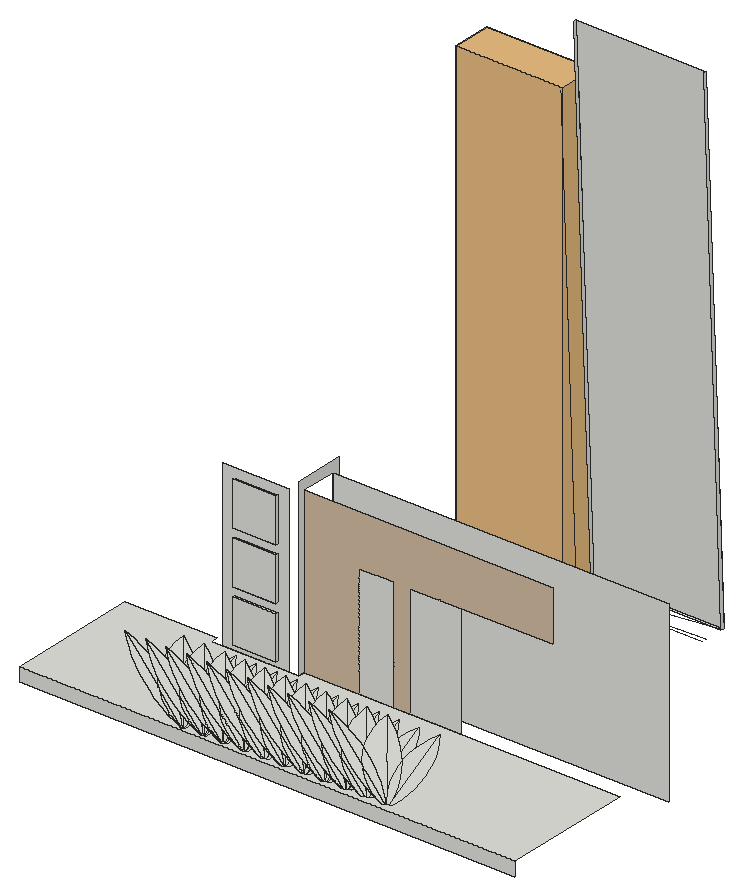
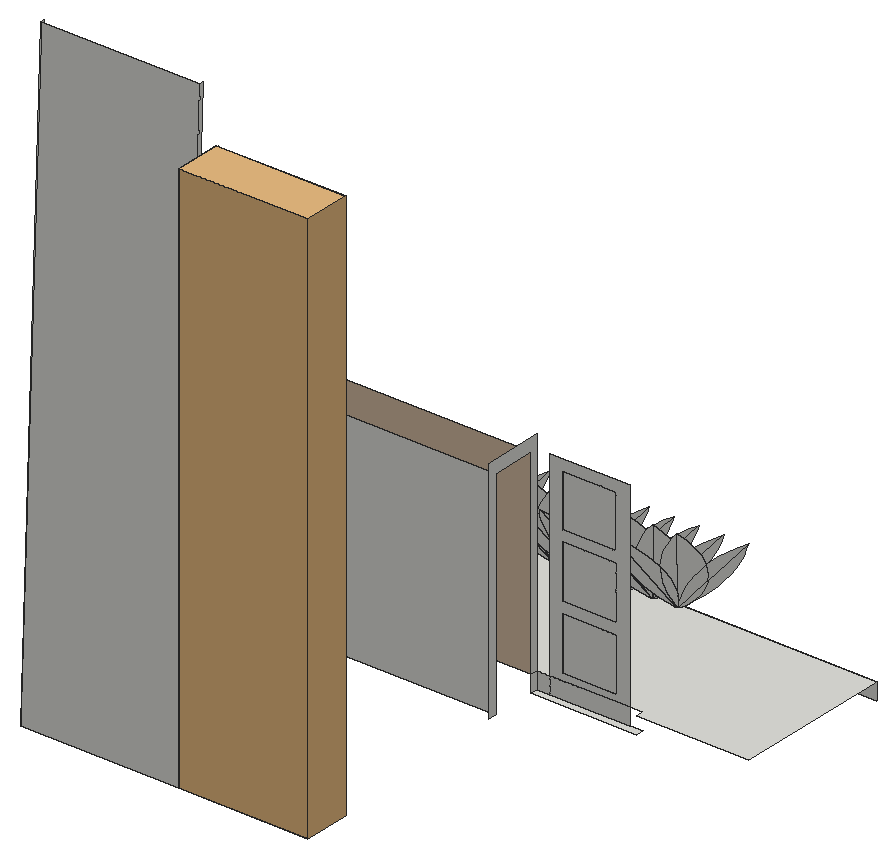
# SketchUp Ruby script. Lengths in inches.
U = 1.inch
M = Sketchup.active_model
def pt(a) = Geom::Point3d.new(a.map { |v| v * U })
def face(e, loops, mat)
  f = e.add_face(loops[0].map { |a| pt(a) })
  loops[1..].each { |l| e.add_face(l.map { |a| pt(a) }).erase! }
  f.material = f.back_material = mat if mat
  f
end
# faces: each face lists its corners as indices into pts; further lists are holes
def faces(e, pts, list, mat = nil) = list.each { |f| face(e, (f[0].is_a?(Array) ? f : [f]).map { |l| l.map { |i| pts[i] } }, mat) }
# xy, xz, yz: faces in a plane at the given z, y or x. An outline is a flat list of corners, or four numbers for a rectangle; further outlines are holes
def ring(l) = l.size == 4 ? [[l[0], l[1]], [l[2], l[1]], [l[2], l[3]], [l[0], l[3]]] : l.each_slice(2).to_a
def flat(e, list, mat, &to3) = list.each { |f| face(e, (f[0].is_a?(Array) ? f : [f]).map { |l| ring(l).map { |u, v| to3.(u, v) } }, mat) }
def xy(e, z, list, mat = nil) = flat(e, list, mat) { |x, y| [x, y, z] }
def xz(e, y, list, mat = nil) = flat(e, list, mat) { |x, z| [x, y, z] }
def yz(e, x, list, mat = nil) = flat(e, list, mat) { |y, z| [x, y, z] }
def lines(e, pts, list) = list.each { |a, b| e.add_line(pt(pts[a]), pt(pts[b])) }
# prism: a flat outline (further loops are holes) pulled along v
def prism(e, loops, v, mat = nil)
  f = face(e, loops, mat); d = Geom::Vector3d.new(v.map { |x| x * U })
  f.pushpull(f.normal.samedirection?(d) ? d.length : -d.length)
end
def box(e, o, s, mat = nil) = prism(e, [[o, [o[0] + s[0], o[1], o[2]], [o[0] + s[0], o[1] + s[1], o[2]], [o[0], o[1] + s[1], o[2]]]], [0, 0, s[2]], mat)
def at(x, y, z, deg = 0) = Geom::Transformation.translation(pt([x, y, z])) * Geom::Transformation.rotation(ORIGIN, Z_AXIS, deg.degrees)
def axes(o, x, y, z) = Geom::Transformation.new([*x, 0, *y, 0, *z, 0, *pt(o).to_a, 1])
def part(name) = M.definitions.add(name)
# library, detail: a bought-in or finely detailed component or shape, given as its bounding box
def library(name, o, s) = part(name).tap { |d| box(d.entities, o, s) }
def detail(e, o, s) = box(e.add_group.entities, o, s)
def put(e, d, t, mat = nil) = e.add_instance(d, t).tap { |i| i.material = mat if mat }
def group(e, t, mat = nil) = e.add_group.tap { |g| g.transformation = t; g.material = mat if mat }.entities
root = M.entities
M.materials.add("[Formica Laminate Light]").color = [213, 189, 164]
xy(root,-6,[[60.83,52.17,96.11,54.73]])
xy(root,-0.3125,[[23.53,1.54,23.53,54.73,60.83,54.73,60.83,52.17,96.11,52.17,96.11,54.73,224.41,54.73,224.41,1.54]])
xy(root,2,[[70.01,51.17,87.63,52.17]])
xy(root,19.625,[[70.01,51.17,87.63,52.17]])
xy(root,23.34,[[70.01,51.17,87.63,52.17]])
xy(root,40.97,[[70.01,51.17,87.63,52.17]])
xy(root,44.6875,[[70.01,51.17,87.63,52.17]])
xz(root,1.54,[[23.53,-6,224.41,-0.3125]])
xz(root,51.17,[[70.01,2,87.63,19.625],[70.01,23.34,87.63,40.97],[70.01,44.6875,87.63,62.3125]])
xz(root,52.17,[[65.07,-6,91.875,-0.3125],[91.875,-6,96.11,-0.3125],[[65.07,-0.3125,91.875,66.01],[70.01,2,87.63,19.625],[70.01,23.34,87.63,40.97],[70.01,44.6875,87.63,62.3125]],[70.01,2,87.63,19.625],[70.01,23.34,87.63,40.97],
  [70.01,44.6875,87.63,62.3125]])
xz(root,54.73,[[118.53,-0.3125,132.41,45.33],[139.125,-0.3125,159.72,45.33]])
xz(root,54.73,[[96.11,-0.3125,118.53,-0.3125,118.53,45.33,132.41,45.33,132.41,-0.3125,139.125,-0.3125,139.125,45.33,196.97,45.33,196.97,66,96.11,66]],"[Formica Laminate Light]")
xz(root,69.27,[[96.11,-6,232.375,66]])
yz(root,87.63,[[51.17,2,52.17,19.625],[51.17,23.34,52.17,40.97],[51.17,44.6875,52.17,62.3125]])
yz(root,96.11,[[52.17,-6,54.73,-0.3125],[69.27,-6,72.34,-6,72.34,70.25,52.17,70.25,52.17,-0.3125,54.73,-0.3125,54.73,66,69.27,66]])
p = [[139.52,3.73,23.55],[138.41,4.22,26.09],[151.99,4.17,10.08],[152.12,4.0625,9.67],[153.32,3.64,7.18],[154.93,3.43,4.77],
  [156.93,3.44,2.47],[159.27,3.67,0.32],[161.95,4.12,-1.66],[159.2,3.65,0.33],[156.59,3.26,2.4],[154.11,2.96,4.54],
  [151.76,2.74,6.74],[149.55,2.62,9],[147.49,2.58,11.3125],[145.58,2.63,13.68],[143.83,2.78,16.09],[142.23,3.01,18.54],
  [140.79,3.33,21.03],[147.66,3.88,23.47],[146.55,4.375,26.01],[160.13,4.32,10],[160.26,4.21,9.59],[161.47,3.79,7.1],
  [163.08,3.58,4.69],[165.07,3.59,2.39],[167.41,3.82,0.24],[170.09,4.27,-1.74],[167.35,3.8,0.25],[164.73,3.41,2.32],
  [162.25,3.11,4.46],[159.9,2.89,6.66],[157.69,2.77,8.92],[155.63,2.73,11.23],[153.72,2.79,13.6],[151.97,2.93,16.01],
  [150.37,3.16,18.46],[148.93,3.48,20.95],[155.62,12.33,26.58],[160.82,5.58,3.36],[160.85,5.38,2.82],[161.26,4.69,0.58],
  [161.04,4.72,0.92],[159.92,5.22,3.48],[158.6,5.6,6.01],[157.08,5.88,8.49],[155.37,6.05,10.93],[153.46,6.12,13.32],
  [151.375,6.07,15.64],[151.02,6.05,16],[151.06,6.57,17.29],[151.57,7.79,19.77],[152.51,9.16,22.16],[153.87,10.68,24.44],
  [150.98,5.54,14.75],[151.33,4.7,12.2],[160.73,6.21,5.07],[160.9,7.17,7.29],[161.36,8.24,9.48],[162.1,9.42,11.61],
  [162.9,10.42,13.23],[163.07,10.25,12.61],[163.49,9.5,10.18],[163.67,8.625,7.76],[163.6,7.65,5.36],[163.29,6.57,2.98],
  [162.74,5.39,0.64],[169.79,16.625,20.93],[172.05,18.25,22.42],[163.12,10.7,13.67],[164.41,12.07,15.65],[165.96,13.52,17.53],
  [167.76,15.04,19.29],[172.36,17.52,20.22],[172.45,16.7,18.02],[172.33,15.78,15.83],[171.99,14.78,13.67],[171.44,13.6875,11.54],
  [170.68,12.52,9.46],[169.72,11.27,7.43],[168.55,9.96,5.45],[167.18,8.58,3.55],[165.62,7.14,1.73],[163.87,5.66,-0.01],
  [159.12,5.69,14.67],[159.16,6.2,15.92],[159.52,6.22,15.5625],[161.61,6.27,13.24],[163.51,6.21,10.85],[165.23,6.03,8.41],
  [166.75,5.75,5.93],[168.06,5.37,3.4],[169.18,4.875,0.84],[159.48,4.85,12.12],[163.76,12.48,26.5],[168.96,5.73,3.28],
  [168.99,5.54,2.75],[169.4,4.84,0.5],[159.2,6.73,17.21],[159.71,7.9375,19.6875],[160.65,9.31,22.08],[162.01,10.84,24.36],
  [168.875,6.36,4.99],[169.04,7.32,7.21],[169.5,8.39,9.4],[170.24,9.57,11.53],[171.04,10.57,13.15],[171.21,10.41,12.53],
  [171.63,9.65,10.1],[171.81,8.78,7.6875],[171.74,7.8,5.28],[171.43,6.72,2.9],[170.88,5.54,0.56],[177.93,16.78,20.85],
  [180.19,18.4,22.34],[171.26,10.85,13.59],[172.55,12.22,15.57],[174.1,13.67,17.45],[175.9,15.19,19.21],[180.5,17.68,20.14],
  [180.59,16.85,17.9375],[180.47,15.9375,15.75],[180.13,14.93,13.59],[179.59,13.84,11.46],[178.83,12.67,9.38],[177.86,11.43,7.35],
  [176.6875,10.11,5.375],[175.32,8.73,3.47],[173.76,7.3,1.65],[172.01,5.81,-0.09],[131.375,3.58,23.625],[130.27,4.07,26.17],
  [143.85,4.01,10.16],[143.98,3.91,9.74],[145.18,3.48,7.26],[146.79,3.28,4.85],[148.78,3.29,2.55],[151.13,3.52,0.4],
  [153.8,3.97,-1.58],[151.0625,3.49,0.41],[148.45,3.11,2.48],[145.96,2.8,4.62],[143.62,2.59,6.82],[141.41,2.47,9.08],
  [139.35,2.43,11.39],[137.4375,2.48,13.76],[135.68,2.625,16.17],[134.09,2.85,18.62],[132.65,3.17,21.11],[142.84,5.39,14.83],
  [142.875,5.9,16.07],[143.23,5.92,15.72],[145.32,5.97,13.4],[147.23,5.9,11.01],[148.94,5.73,8.57],[150.46,5.45,6.08],
  [151.78,5.0625,3.56],[152.9,4.57,1],[143.19,4.55,12.28],[147.48,12.18,26.65],[152.68,5.43,3.4375],[152.71,5.23,2.9],
  [153.11,4.53,0.66],[142.92,6.42,17.37],[143.43,7.64,19.85],[144.37,9.01,22.24],[145.72,10.53,24.52],[152.59,6.0625,5.15],
  [152.76,7.01,7.37],[153.22,8.09,9.56],[153.96,9.27,11.6875],[154.76,10.27,13.31],[154.93,10.1,12.68],[155.35,9.34,10.26],
  [155.52,8.47,7.84],[155.46,7.5,5.44],[155.15,6.42,3.06],[154.6,5.24,0.72],[161.65,16.47,21],[163.91,18.1,22.5],
  [154.97,10.55,13.75],[156.26,11.92,15.73],[157.8125,13.37,17.6],[159.61,14.89,19.37],[164.21,17.37,20.3],[164.31,16.55,18.1],
  [164.1875,15.63,15.91],[163.85,14.625,13.75],[163.3,13.54,11.62],[162.54,12.37,9.54],[161.57,11.12,7.5],[160.4,9.81,5.53],
  [159.04,8.43,3.63],[157.48,6.99,1.81],[155.73,5.5,0.07],[123.23,3.43,23.7],[122.13,3.92,26.25],[135.71,3.86,10.24],
  [135.84,3.76,9.82],[137.04,3.33,7.34],[138.65,3.125,4.93],[140.64,3.14,2.63],[142.99,3.37,0.48],[145.66,3.82,-1.5],
  [142.92,3.34,0.49],[140.31,2.95,2.56],[137.82,2.65,4.69],[135.47,2.4375,6.89],[133.27,2.3125,9.15],[131.21,2.28,11.47],
  [129.3,2.33,13.84],[127.54,2.47,16.25],[125.94,2.7,18.7],[124.51,3.02,21.1875],[139.33,12.03,26.73],[144.54,5.28,3.52],
  [144.57,5.08,2.98],[144.97,4.38,0.73],[144.75,4.42,1.08],[143.64,4.91,3.64],[142.32,5.3,6.16],[140.8,5.58,8.65],
  [139.08,5.75,11.09],[137.18,5.8125,13.48],[135.09,5.77,15.8],[134.73,5.74,16.15],[134.78,6.27,17.44],[135.29,7.48,19.93],
  [136.23,8.86,22.32],[137.58,10.38,24.6],[134.7,5.24,14.91],[135.05,4.4,12.36],[144.45,5.91,5.23],[144.62,6.86,7.45],
  [145.07,7.93,9.64],[145.8125,9.11,11.77],[146.61,10.12,13.39],[146.78,9.95,12.76],[147.21,9.19,10.34],[147.38,8.32,7.92],
  [147.32,7.34,5.52],[147.01,6.26,3.14],[146.45,5.09,0.8],[153.51,16.32,21.08],[155.76,17.95,22.58],[146.83,10.39,13.83],
  [148.12,11.77,15.81],[149.67,13.22,17.68],[151.47,14.74,19.45],[156.07,17.22,20.375],[156.17,16.4,18.17],[156.04,15.48,15.99],
  [155.71,14.48,13.83],[155.16,13.39,11.7],[154.4,12.22,9.62],[153.43,10.97,7.58],[152.26,9.66,5.61],[150.89,8.28,3.71],
  [149.33,6.84,1.89],[147.59,5.35,0.15],[115.09,3.28,23.78],[113.99,3.77,26.33],[127.57,3.71,10.3125],[127.69,3.61,9.9],
  [128.9,3.18,7.41],[130.51,2.97,5.01],[132.5,2.99,2.71],[134.85,3.22,0.56],[137.52,3.67,-1.42],[134.78,3.19,0.57],
  [132.16,2.8,2.64],[129.68,2.5,4.77],[127.33,2.29,6.97],[125.125,2.16,9.23],[123.07,2.125,11.55],[121.16,2.18,13.92],
  [119.4,2.32,16.33],[117.8,2.55,18.78],[116.37,2.87,21.27],[131.19,11.875,26.8125],[136.4,5.125,3.6],[136.42,4.93,3.0625],
  [136.83,4.23,0.8125],[136.61,4.27,1.16],[135.5,4.76,3.72],[134.18,5.15,6.24],[132.66,5.43,8.73],[130.94,5.6,11.17],
  [129.04,5.66,13.55],[126.95,5.62,15.88],[126.59,5.59,16.23],[126.63,6.12,17.52],[127.15,7.33,20],[128.09,8.71,22.4],
  [129.44,10.23,24.68],[126.55,5.09,14.99],[126.91,4.24,12.44],[136.31,5.76,5.31],[136.48,6.71,7.53],[136.93,7.78,9.72],
  [137.67,8.96,11.85],[138.47,9.97,13.46],[138.64,9.8,12.84],[139.0625,9.04,10.42],[139.24,8.17,8],[139.17,7.19,5.6],
  [138.86,6.11,3.22],[138.3125,4.9375,0.875],[145.37,16.17,21.16],[147.62,17.8,22.66],[138.69,10.24,13.91],[139.98,11.61,15.89],
  [141.53,13.07,17.76],[143.33,14.59,19.53],[147.93,17.07,20.45],[148.02,16.24,18.25],[147.9,15.33,16.07],[147.57,14.32,13.91],
  [147.02,13.23,11.78],[146.26,12.0625,9.7],[145.29,10.82,7.66],[144.12,9.5,5.69],[142.75,8.125,3.79],[141.19,6.6875,1.96],
  [139.45,5.2,0.23],[98.81,2.97,23.94],[97.7,3.46,26.48],[111.28,3.41,10.47],[111.41,3.3,10.0625],[112.62,2.88,7.57],
  [114.22,2.67,5.17],[116.22,2.68,2.87],[118.5625,2.91,0.72],[121.24,3.36,-1.26],[118.5,2.89,0.73],[115.88,2.5,2.8],
  [113.4,2.2,4.93],[111.05,1.98,7.13],[108.84,1.86,9.39],[106.78,1.82,11.71],[104.87,1.875,14.07],[103.12,2.02,16.49],
  [101.52,2.25,18.9375],[100.08,2.57,21.42],[106.95,3.125,23.86],[105.85,3.62,26.41],[119.42,3.56,10.39],[119.55,3.45,9.98],
  [120.76,3.03,7.49],[122.37,2.82,5.09],[124.36,2.83,2.79],[126.71,3.07,0.64],[129.38,3.52,-1.34],[126.64,3.04,0.65],
  [124.02,2.65,2.72],[121.54,2.35,4.85],[119.19,2.13,7.05],[116.98,2.01,9.3125],[114.92,1.97,11.63],[113.01,2.03,13.99],
  [111.26,2.17,16.41],[109.66,2.4,18.86],[108.22,2.72,21.35],[114.91,11.57,26.97],[120.11,4.82,3.75],[120.14,4.625,3.22],
  [120.55,3.93,0.97],[120.33,3.96,1.32],[119.21,4.46,3.875],[117.89,4.84,6.4],[116.375,5.125,8.89],[114.66,5.3,11.33],
  [112.75,5.36,13.71],[110.67,5.3125,16.04],[110.31,5.29,16.39],[110.35,5.82,17.68],[110.86,7.03,20.16],[111.8,8.4,22.56],
  [113.16,9.92,24.84],[110.27,4.78,15.15],[110.625,3.94,12.6],[120.02,5.45,5.47],[120.19,6.41,7.6875],[120.65,7.48,9.875],
  [121.39,8.66,12.01],[122.1875,9.66,13.62],[122.36,9.5,13],[122.78,8.74,10.58],[122.96,7.87,8.16],[122.89,6.89,5.76],
  [122.58,5.81,3.375],[122.03,4.63,1.03],[129.08,15.86,21.32],[131.34,17.49,22.82],[122.41,9.9375,14.07],[123.7,11.31,16.04],
  [125.25,12.76,17.92],[127.05,14.28,19.69],[131.65,16.76,20.61],[131.74,15.94,18.41],[131.62,15.02,16.23],[131.28,14.02,14.07],
  [130.73,12.93,11.9375],[129.97,11.76,9.85],[129.01,10.51,7.82],[127.84,9.2,5.85],[126.47,7.82,3.95],[124.91,6.39,2.125],
  [123.16,4.9,0.38],[118.41,4.93,15.07],[118.45,5.44,16.3125],[118.81,5.46,15.96],[120.9,5.51,13.63],[122.8,5.45,11.25],
  [124.52,5.28,8.81],[126.04,5,6.32],[127.35,4.61,3.8],[128.47,4.11,1.24],[118.77,4.09,12.52],[123.05,11.72,26.89],
  [128.25,4.97,3.68],[128.28,4.78,3.14],[128.6875,4.08,0.89],[118.49,5.97,17.6],[119,7.18,20.08],[119.94,8.56,22.48],
  [121.3,10.08,24.76],[128.16,5.61,5.39],[128.33,6.56,7.61],[128.79,7.63,9.79],[129.53,8.81,11.93],[130.33,9.8125,13.54],
  [130.5,9.65,12.92],[130.92,8.89,10.5],[131.1,8.02,8.08],[131.03,7.04,5.68],[130.72,5.96,3.3],[130.17,4.78,0.95],
  [137.22,16.02,21.24],[139.48,17.64,22.74],[130.55,10.09,13.99],[131.84,11.46,15.97],[133.39,12.91,17.84],[135.1875,14.44,19.61],
  [139.79,16.92,20.53],[139.88,16.09,18.33],[139.76,15.18,16.15],[139.42,14.17,13.99],[138.875,13.08,11.86],[138.12,11.91,9.77],
  [137.15,10.67,7.74],[135.98,9.35,5.77],[134.61,7.97,3.87],[133.05,6.54,2.04],[131.3,5.05,0.3],[90.67,2.82,24.02],
  [89.5625,3.3125,26.5625],[103.14,3.25,10.55],[103.27,3.15,10.14],[104.47,2.73,7.65],[106.08,2.52,5.24],[108.07,2.53,2.95],
  [110.42,2.76,0.8],[113.09,3.21,-1.18],[110.35,2.74,0.81],[107.74,2.35,2.875],[105.25,2.04,5.01],[102.91,1.83,7.21],
  [100.7,1.71,9.47],[98.64,1.67,11.79],[96.73,1.72,14.15],[94.97,1.87,16.5625],[93.375,2.1,19.02],[91.9375,2.41,21.5],
  [102.13,4.63,15.23],[102.17,5.14,16.47],[102.52,5.16,16.12],[104.61,5.21,13.79],[106.52,5.14,11.41],[108.23,4.97,8.97],
  [109.75,4.69,6.48],[111.07,4.3,3.95],[112.1875,3.81,1.4],[102.48,3.79,12.68],[106.77,11.42,27.05],[111.97,4.67,3.83],
  [112,4.47,3.3],[112.4,3.77,1.05],[102.21,5.66,17.76],[102.72,6.875,20.24],[103.66,8.25,22.64],[105.02,9.77,24.92],
  [111.88,5.3,5.54],[112.05,6.26,7.77],[112.51,7.33,9.95],[113.25,8.51,12.08],[114.05,9.51,13.7],[114.22,9.34,13.08],
  [114.64,8.58,10.66],[114.82,7.71,8.24],[114.75,6.74,5.84],[114.4375,5.66,3.46],[113.89,4.48,1.11],[120.94,15.71,21.4],
  [123.2,17.34,22.9],[114.27,9.79,14.15],[115.55,11.16,16.125],[117.1,12.61,18],[118.9,14.13,19.76],[123.5,16.61,20.69],
  [123.6,15.79,18.49],[123.48,14.875,16.31],[123.14,13.87,14.14],[122.59,12.78,12.02],[121.83,11.61,9.93],[120.87,10.36,7.9],
  [119.7,9.05,5.93],[118.33,7.67,4.03],[116.77,6.23,2.2],[115.02,4.75,0.46],[82.52,2.67,24.1],[81.42,3.16,26.64],
  [95,3.1,10.63],[95.125,3,10.22],[96.33,2.57,7.73],[97.94,2.37,5.32],[99.93,2.38,3.03],[102.28,2.61,0.875],
  [104.95,3.06,-1.1],[102.21,2.58,0.89],[99.6,2.19,2.96],[97.11,1.89,5.09],[94.76,1.68,7.29],[92.56,1.55,9.55],
  [90.5,1.52,11.87],[88.59,1.57,14.23],[86.83,1.71,16.64],[85.23,1.94,19.1],[83.8,2.26,21.58],[98.625,11.27,27.13],
  [103.83,4.52,3.91],[103.86,4.32,3.38],[104.26,3.62,1.13],[104.04,3.66,1.48],[102.93,4.15,4.03],[101.61,4.54,6.56],
  [100.09,4.82,9.05],[98.375,4.99,11.49],[96.47,5.06,13.87],[94.38,5.01,16.2],[94.02,4.98,16.55],[94.07,5.51,17.84],
  [94.58,6.72,20.32],[95.52,8.1,22.72],[96.875,9.62,25],[93.99,4.48,15.31],[94.34,3.64,12.76],[103.74,5.15,5.625],
  [103.91,6.1,7.85],[104.36,7.17,10.03],[105.1,8.35,12.16],[105.9,9.36,13.78],[106.07,9.19,13.16],[106.5,8.43,10.74],
  [106.67,7.5625,8.32],[106.61,6.58,5.91],[106.3,5.51,3.54],[105.74,4.33,1.19],[112.8,15.5625,21.48],[115.05,17.1875,22.98],
  [106.125,9.63,14.23],[107.41,11.01,16.2],[108.96,12.46,18.08],[110.76,13.98,19.84],[115.36,16.46,20.77],[115.46,15.64,18.57],
  [115.33,14.72,16.38],[115,13.72,14.22],[114.45,12.625,12.1],[113.69,11.46,10.01],[112.72,10.21,7.98],[111.55,8.9,6.01],
  [110.18,7.52,4.11],[108.625,6.08,2.28],[106.88,4.59,0.54],[74.38,2.52,24.18],[73.28,3.01,26.72],[86.86,2.95,10.71],
  [86.98,2.85,10.3],[88.1875,2.42,7.8125],[89.8,2.21,5.4],[91.79,2.23,3.11],[94.14,2.46,0.96],[96.8125,2.91,-1.03],
  [94.07,2.43,0.97],[91.45,2.04,3.03],[88.97,1.74,5.17],[86.62,1.53,7.37],[84.42,1.4,9.63],[82.36,1.37,11.95],
  [80.45,1.42,14.3125],[78.69,1.5625,16.72],[77.09,1.79,19.17],[75.66,2.11,21.66],[85.84,4.33,15.39],[85.88,4.83,16.63],
  [86.24,4.86,16.27],[88.33,4.9,13.95],[90.23,4.84,11.57],[91.95,4.67,9.125],[93.47,4.39,6.64],[94.79,4,4.11],
  [95.9,3.51,1.56],[86.2,3.49,12.84],[90.48,11.11,27.21],[95.6875,4.37,3.99],[95.71,4.17,3.46],[96.12,3.47,1.21],
  [85.92,5.36,17.92],[86.4375,6.57,20.4],[87.375,7.95,22.8],[88.73,9.47,25.08],[95.6,5,5.7],[95.77,5.95,7.93],
  [96.22,7.02,10.11],[96.96,8.2,12.24],[97.76,9.21,13.86],[97.93,9.04,13.24],[98.35,8.28,10.82],[98.53,7.41,8.4],
  [98.47,6.43,5.99],[98.16,5.35,3.61],[97.6,4.18,1.27],[104.66,15.41,21.56],[106.91,17.04,23.06],[97.98,9.48,14.31],
  [99.27,10.85,16.28],[100.82,12.31,18.16],[102.62,13.83,19.92],[107.22,16.31,20.85],[107.3125,15.49,18.65],[107.19,14.57,16.46],
  [106.86,13.5625,14.3],[106.31,12.47,12.18],[105.55,11.3,10.09],[104.58,10.06,8.06],[103.41,8.74,6.09],[102.04,7.37,4.1875],
  [100.48,5.93,2.36],[98.74,4.44,0.62],[66.24,2.36,24.26],[65.14,2.86,26.8],[78.72,2.8,10.79],[78.84,2.7,10.38],
  [80.05,2.27,7.89],[81.66,2.0625,5.48],[83.65,2.07,3.1875],[86,2.31,1.03],[88.67,2.76,-0.95],[85.93,2.28,1.05],
  [83.3125,1.89,3.11],[80.83,1.59,5.25],[78.48,1.375,7.45],[76.27,1.25,9.71],[74.21,1.21,12.02],[72.3,1.27,14.39],
  [70.55,1.41,16.8],[68.95,1.64,19.25],[67.51,1.96,21.74],[82.34,10.96,27.29],[87.54,4.21,4.07],[87.57,4.02,3.54],
  [87.98,3.32,1.29],[87.76,3.35,1.63],[86.65,3.85,4.19],[85.33,4.24,6.72],[83.81,4.52,9.21],[82.09,4.6875,11.64],
  [80.1875,4.75,14.03],[78.1,4.71,16.35],[77.74,4.68,16.71],[77.78,5.21,18],[78.29,6.42,20.48],[79.23,7.8,22.875],
  [80.59,9.32,25.16],[77.7,4.17,15.47],[78.06,3.33,12.92],[87.45,4.85,5.78],[87.625,5.8,8.01],[88.08,6.87,10.19],
  [88.82,8.05,12.32],[89.62,9.05,13.94],[89.79,8.89,13.32],[90.21,8.13,10.9],[90.39,7.26,8.48],[90.32,6.28,6.07],
  [90.01,5.2,3.69],[89.46,4.02,1.35],[96.51,15.26,21.64],[98.77,16.88,23.14],[89.84,9.33,14.38],[91.13,10.7,16.36],
  [92.68,12.15,18.24],[94.48,13.68,20],[99.08,16.16,20.93],[99.17,15.33,18.73],[99.05,14.42,16.54],[98.71,13.41,14.38],
  [98.17,12.32,12.26],[97.41,11.15,10.17],[96.4375,9.91,8.14],[95.27,8.59,6.17],[93.9,7.21,4.27],[92.34,5.78,2.44],
  [90.59,4.29,0.7],[170.55,11.05,14.9375],[165.5625,12.44,24.29],[167.15,12.28,22.02],[168.51,11.99,19.7],[169.65,11.58,17.33],
  [154.26,10.75,15.1],[149.28,12.14,24.45],[150.86,11.97,22.18],[152.23,11.69,19.85],[153.36,11.28,17.49],[162.41,10.9,15.02],
  [157.42,12.29,24.37],[159.01,12.125,22.1],[160.37,11.84,19.78],[161.5,11.43,17.41],[146.12,10.6,15.18],[141.14,11.98,24.53],
  [142.72,11.82,22.26],[144.09,11.53,19.93],[145.22,11.125,17.57],[137.98,10.44,15.26],[132.99,11.83,24.61],[134.58,11.67,22.34],
  [135.94,11.38,20.01],[137.08,10.97,17.65],[129.84,10.29,15.34],[124.85,11.68,24.68],[126.4375,11.52,22.41],[127.8,11.23,20.09],
  [128.9375,10.82,17.73],[113.55,9.99,15.49],[108.57,11.38,24.84],[110.15,11.21,22.57],[111.52,10.93,20.25],[112.65,10.52,17.89],
  [121.7,10.14,15.41],[116.71,11.53,24.76],[118.3,11.37,22.49],[119.66,11.08,20.17],[120.79,10.67,17.81],[105.41,9.84,15.57],
  [100.43,11.23,24.92],[102.01,11.0625,22.65],[103.375,10.77,20.33],[104.51,10.37,17.97],[97.27,9.6875,15.65],[92.28,11.07,25],
  [93.87,10.91,22.73],[95.23,10.62,20.41],[96.37,10.21,18.05],[89.13,9.53,15.73],[84.14,10.92,25.08],[85.73,10.76,22.8125],
  [87.09,10.47,20.49],[88.23,10.0625,18.125],[149.46,4.96,24.1],[152.21,5.44,22.09],[154.8125,5.81,19.99],[157.25,6.07,17.82],
  [141.32,4.81,24.18],[144.07,5.28,22.17],[146.67,5.65,20.07],[149.11,5.92,17.9],[125.03,4.5,24.34],[127.79,4.98,22.33],
  [130.39,5.35,20.23],[132.82,5.61,18.05],[133.17,4.65,24.26],[135.93,5.13,22.25],[138.53,5.5,20.15],[140.97,5.77,17.97],
  [116.89,4.35,24.41],[119.64,4.83,22.41],[122.25,5.2,20.3125],[124.68,5.46,18.13],[108.75,4.2,24.49],[111.5,4.68,22.49],
  [114.1,5.05,20.39],[116.54,5.31,18.21],[100.61,4.05,24.57],[103.36,4.52,22.57],[105.96,4.89,20.47],[108.4,5.16,18.29],
  [84.32,3.74,24.73],[87.08,4.22,22.72],[89.68,4.59,20.63],[92.11,4.85,18.45],[92.46,3.9,24.65],[95.22,4.37,22.65],
  [97.82,4.74,20.55],[100.26,5.01,18.37],[76.18,3.59,24.8125],[78.94,4.07,22.8],[81.54,4.4375,20.71],[83.97,4.7,18.53],
  [68.04,3.44,24.89],[70.79,3.92,22.88],[73.39,4.29,20.79],[75.83,4.55,18.61],[134.88,148.73,0],[182.53,150.73,0],
  [182.53,158.26,0.32],[129.74,150.73,0],[129.74,142.91,184.48],[182.53,148.73,0]]
faces(root,p,[[0,1,2,3,4,5,6,7,8,9,10,11,12,13,14,15,16,17,18],[19,20,21,22,23,24,25,26,27,28,29,30,31,32,33,34,35,36,37],[3,2,8,7,6,5,4],[22,21,27,26,25,24,23],[38,39,40,41,8,42,43,44,45,46,47,48,49,50,51,52,53],[54,49,48,47,46,45,44,43,42,8,2,55],[8,39,56,57,58,59,60,61,62,63,64,65,66],[39,8,41,40],
  [67,68,8,66,65,64,63,62,61,60,69,70,71,72],[8,68,73,74,75,76,77,78,79,80,81,82,83],[84,85,86,87,88,89,90,91,92,27,21,93],[94,95,96,97,27,92,91,90,89,88,87,86,85,98,99,100,101],[27,95,102,103,104,105,106,107,108,109,110,111,112],[95,27,97,96],[113,114,27,112,111,110,109,108,107,106,115,116,117,118],[27,114,119,120,121,122,123,124,125,126,127,128,129],
  [130,131,132,133,134,135,136,137,138,139,140,141,142,143,144,145,146,147,148],[133,132,138,137,136,135,134],[149,150,151,152,153,154,155,156,157,138,132,158],[159,160,161,162,138,157,156,155,154,153,152,151,150,163,164,165,166],[138,160,167,168,169,170,171,172,173,174,175,176,177],[160,138,162,161],[178,179,138,177,176,175,174,173,172,171,180,181,182,183],[138,179,184,185,186,187,188,189,190,191,192,193,194],
  [195,196,197,198,199,200,201,202,203,204,205,206,207,208,209,210,211,212,213],[198,197,203,202,201,200,199],[214,215,216,217,203,218,219,220,221,222,223,224,225,226,227,228,229],[230,225,224,223,222,221,220,219,218,203,197,231],[203,215,232,233,234,235,236,237,238,239,240,241,242],[215,203,217,216],[243,244,203,242,241,240,239,238,237,236,245,246,247,248],[203,244,249,250,251,252,253,254,255,256,257,258,259],
  [260,261,262,263,264,265,266,267,268,269,270,271,272,273,274,275,276,277,278],[263,262,268,267,266,265,264],[279,280,281,282,268,283,284,285,286,287,288,289,290,291,292,293,294],[295,290,289,288,287,286,285,284,283,268,262,296],[268,280,297,298,299,300,301,302,303,304,305,306,307],[280,268,282,281],[308,309,268,307,306,305,304,303,302,301,310,311,312,313],[268,309,314,315,316,317,318,319,320,321,322,323,324],
  [325,326,327,328,329,330,331,332,333,334,335,336,337,338,339,340,341,342,343],[344,345,346,347,348,349,350,351,352,353,354,355,356,357,358,359,360,361,362],[328,327,333,332,331,330,329],[347,346,352,351,350,349,348],[363,364,365,366,333,367,368,369,370,371,372,373,374,375,376,377,378],[379,374,373,372,371,370,369,368,367,333,327,380],[333,364,381,382,383,384,385,386,387,388,389,390,391],[364,333,366,365],
  [392,393,333,391,390,389,388,387,386,385,394,395,396,397],[333,393,398,399,400,401,402,403,404,405,406,407,408],[409,410,411,412,413,414,415,416,417,352,346,418],[419,420,421,422,352,417,416,415,414,413,412,411,410,423,424,425,426],[352,420,427,428,429,430,431,432,433,434,435,436,437],[420,352,422,421],[438,439,352,437,436,435,434,433,432,431,440,441,442,443],[352,439,444,445,446,447,448,449,450,451,452,453,454],
  [455,456,457,458,459,460,461,462,463,464,465,466,467,468,469,470,471,472,473],[458,457,463,462,461,460,459],[474,475,476,477,478,479,480,481,482,463,457,483],[484,485,486,487,463,482,481,480,479,478,477,476,475,488,489,490,491],[463,485,492,493,494,495,496,497,498,499,500,501,502],[485,463,487,486],[503,504,463,502,501,500,499,498,497,496,505,506,507,508],[463,504,509,510,511,512,513,514,515,516,517,518,519],
  [520,521,522,523,524,525,526,527,528,529,530,531,532,533,534,535,536,537,538],[523,522,528,527,526,525,524],[539,540,541,542,528,543,544,545,546,547,548,549,550,551,552,553,554],[555,550,549,548,547,546,545,544,543,528,522,556],[528,540,557,558,559,560,561,562,563,564,565,566,567],[540,528,542,541],[568,569,528,567,566,565,564,563,562,561,570,571,572,573],[528,569,574,575,576,577,578,579,580,581,582,583,584],
  [585,586,587,588,589,590,591,592,593,594,595,596,597,598,599,600,601,602,603],[588,587,593,592,591,590,589],[604,605,606,607,608,609,610,611,612,593,587,613],[614,615,616,617,593,612,611,610,609,608,607,606,605,618,619,620,621],[593,615,622,623,624,625,626,627,628,629,630,631,632],[615,593,617,616],[633,634,593,632,631,630,629,628,627,626,635,636,637,638],[593,634,639,640,641,642,643,644,645,646,647,648,649],
  [650,651,652,653,654,655,656,657,658,659,660,661,662,663,664,665,666,667,668],[653,652,658,657,656,655,654],[669,670,671,672,658,673,674,675,676,677,678,679,680,681,682,683,684],[685,680,679,678,677,676,675,674,673,658,652,686],[670,658,672,671],[658,670,687,688,689,690,691,692,693,694,695,696,697],[698,699,658,697,696,695,694,693,692,691,700,701,702,703],[658,699,704,705,706,707,708,709,710,711,712,713,714],
  [715,106,105,104,103,102,95,94,716,717,718,719],[720,171,170,169,168,167,160,159,721,722,723,724],[725,60,59,58,57,56,39,38,726,727,728,729],[730,236,235,234,233,232,215,214,731,732,733,734],[735,301,300,299,298,297,280,279,736,737,738,739],[740,431,430,429,428,427,420,419,741,742,743,744],[745,496,495,494,493,492,485,484,746,747,748,749],[750,385,384,383,382,381,364,363,751,752,753,754],
  [755,561,560,559,558,557,540,539,756,757,758,759],[760,626,625,624,623,622,615,614,761,762,763,764],[765,691,690,689,688,687,670,669,766,767,768,769],[21,20,770,771,772,773,85,84,93],[2,1,774,775,776,777,49,54,55],[197,196,778,779,780,781,225,230,231],[132,131,782,783,784,785,150,149,158],[262,261,786,787,788,789,290,295,296],
  [346,345,790,791,792,793,410,409,418],[327,326,794,795,796,797,374,379,380],[522,521,798,799,800,801,550,555,556],[457,456,802,803,804,805,475,474,483],[587,586,806,807,808,809,605,604,613],[652,651,810,811,812,813,680,685,686]])
lines(root,p,[[814,815],[816,817],[817,818],[814,819]])
detail(root,[86.53,143.85,0],[43.21,15.63,184.95])
g1 = group(root,at(129.74,150.73,0))
yz(g1,0,[[7.54,-0.05,-1.21,206.28,0,206.33,8.75,0]])
yz(g1,52.79,[[7.54,-0.05,8.75,0,0,206.33,-1.21,206.28]])
p = [[0,8.75,0],[52.79,8.75,0],[52.79,7.54,-0.05],[0,7.54,-0.05],[0,0,206.33],[52.79,0,206.33]]
faces(g1,p,[[0,1,2,3],[0,4,5,1]])
